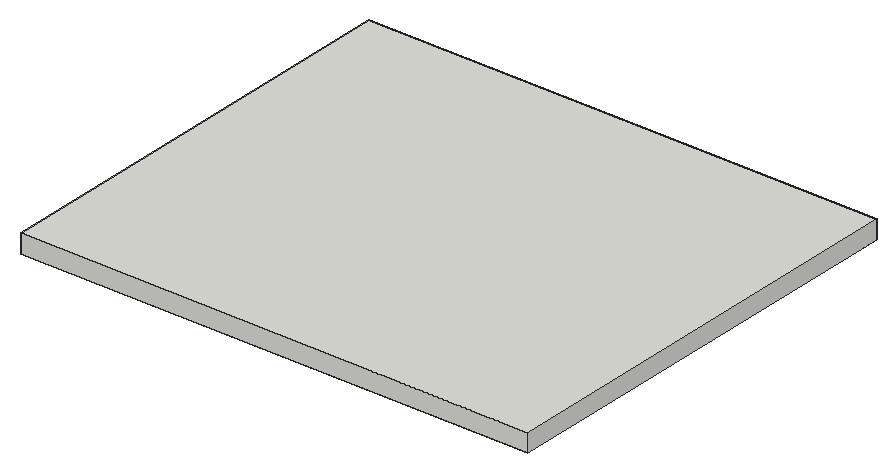
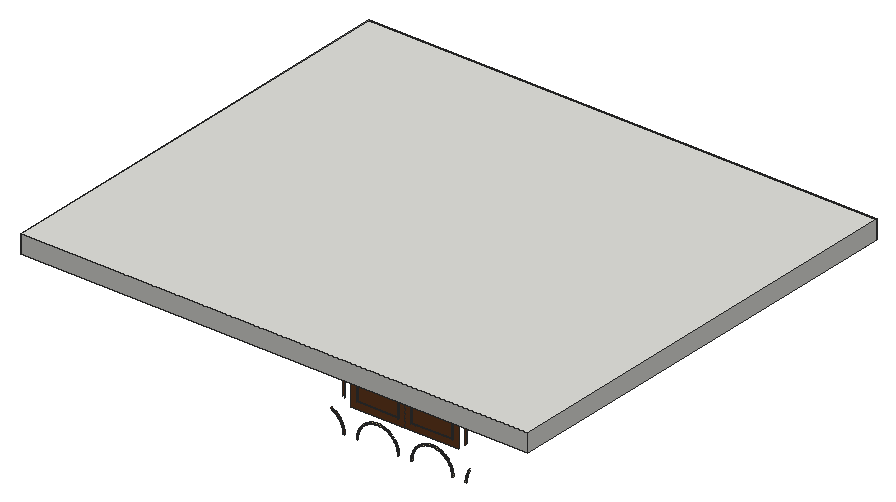
# SketchUp Ruby script. Lengths in inches.
U = 1.inch
M = Sketchup.active_model
def pt(a) = Geom::Point3d.new(a.map { |v| v * U })
def face(e, loops, mat)
  f = e.add_face(loops[0].map { |a| pt(a) })
  loops[1..].each { |l| e.add_face(l.map { |a| pt(a) }).erase! }
  f.material = f.back_material = mat if mat
  f
end
# faces: each face lists its corners as indices into pts; further lists are holes
def faces(e, pts, list, mat = nil) = list.each { |f| face(e, (f[0].is_a?(Array) ? f : [f]).map { |l| l.map { |i| pts[i] } }, mat) }
# xy, xz, yz: faces in a plane at the given z, y or x. An outline is a flat list of corners, or four numbers for a rectangle; further outlines are holes
def ring(l) = l.size == 4 ? [[l[0], l[1]], [l[2], l[1]], [l[2], l[3]], [l[0], l[3]]] : l.each_slice(2).to_a
def flat(e, list, mat, &to3) = list.each { |f| face(e, (f[0].is_a?(Array) ? f : [f]).map { |l| ring(l).map { |u, v| to3.(u, v) } }, mat) }
def xy(e, z, list, mat = nil) = flat(e, list, mat) { |x, y| [x, y, z] }
def xz(e, y, list, mat = nil) = flat(e, list, mat) { |x, z| [x, y, z] }
def yz(e, x, list, mat = nil) = flat(e, list, mat) { |y, z| [x, y, z] }
def lines(e, pts, list) = list.each { |a, b| e.add_line(pt(pts[a]), pt(pts[b])) }
# prism: a flat outline (further loops are holes) pulled along v
def prism(e, loops, v, mat = nil)
  f = face(e, loops, mat); d = Geom::Vector3d.new(v.map { |x| x * U })
  f.pushpull(f.normal.samedirection?(d) ? d.length : -d.length)
end
def box(e, o, s, mat = nil) = prism(e, [[o, [o[0] + s[0], o[1], o[2]], [o[0] + s[0], o[1] + s[1], o[2]], [o[0], o[1] + s[1], o[2]]]], [0, 0, s[2]], mat)
def at(x, y, z, deg = 0) = Geom::Transformation.translation(pt([x, y, z])) * Geom::Transformation.rotation(ORIGIN, Z_AXIS, deg.degrees)
def axes(o, x, y, z) = Geom::Transformation.new([*x, 0, *y, 0, *z, 0, *pt(o).to_a, 1])
def part(name) = M.definitions.add(name)
# library, detail: a bought-in or finely detailed component or shape, given as its bounding box
def library(name, o, s) = part(name).tap { |d| box(d.entities, o, s) }
def detail(e, o, s) = box(e.add_group.entities, o, s)
def put(e, d, t, mat = nil) = e.add_instance(d, t).tap { |i| i.material = mat if mat }
def group(e, t, mat = nil) = e.add_group.tap { |g| g.transformation = t; g.material = mat if mat }.entities
root = M.entities
M.materials.add("138_plaster painted wall texture-seamless").color = [214, 198, 153]
M.materials.add("[Wood Veneer 01]").color = [104, 60, 32]
c1 = part("Recessed ceiling light")
xy(c1.entities,0,[[4,0,2.96,0.14,2,0.54,1.17,1.17,0.54,2,0.14,2.96,0,4,0.14,5.04,0.54,6,1.17,6.83,2,7.46,2.96,7.86,4,8,5.04,7.86,6,7.46,6.83,6.83,7.46,6,7.86,5.04,8,4,7.86,2.96,7.46,2,6.83,1.17,6,0.54,5.04,0.14]])
xy(c1.entities,0.2,[[[4,0,5.04,0.14,6,0.54,6.83,1.17,7.46,2,7.86,2.96,8,4,7.86,5.04,7.46,6,6.83,6.83,6,7.46,5.04,7.86,4,8,2.96,7.86,2,7.46,1.17,6.83,0.54,6,0.14,5.04,0,4,0.14,2.96,0.54,2,1.17,1.17,2,0.54,2.96,0.14],[4,0.6,3.12,0.72,2.3,1.06,1.6,1.6,1.06,2.3,0.72,3.12,0.6,4,0.72,4.88,1.06,5.7,1.6,6.4,2.3,6.94,3.12,7.28,4,7.4,4.88,7.28,5.7,6.94,6.4,6.4,6.94,5.7,7.28,4.88,7.4,4,7.28,3.12,6.94,2.3,6.4,1.6,5.7,1.06,4.88,0.72]],[4,0.6,4.88,0.72,5.7,1.06,6.4,1.6,6.94,2.3,7.28,3.12,7.4,4,7.28,4.88,6.94,5.7,6.4,6.4,5.7,6.94,4.88,7.28,4,7.4,3.12,7.28,2.3,6.94,1.6,6.4,1.06,5.7,0.72,4.88,0.6,4,0.72,3.12,1.06,2.3,1.6,1.6,2.3,1.06,3.12,0.72]])
p = [[2.96,0.14,0],[4,0,0],[4,0,0.2],[2.96,0.14,0.2],[5.04,0.14,0],[5.04,0.14,0.2],
  [2,0.54,0],[2,0.54,0.2],[6,0.54,0],[6,0.54,0.2],[1.17,1.17,0],[1.17,1.17,0.2],
  [6.83,1.17,0],[6.83,1.17,0.2],[0.54,2,0],[0.54,2,0.2],[7.46,2,0],[7.46,2,0.2],
  [0.14,2.96,0],[0.14,2.96,0.2],[7.86,2.96,0],[7.86,2.96,0.2],[0,4,0],[0,4,0.2],
  [8,4,0],[8,4,0.2],[0.14,5.04,0],[0.14,5.04,0.2],[7.86,5.04,0],[7.86,5.04,0.2],
  [0.54,6,0],[0.54,6,0.2],[7.46,6,0],[7.46,6,0.2],[1.17,6.83,0],[1.17,6.83,0.2],
  [6.83,6.83,0],[6.83,6.83,0.2],[2,7.46,0],[2,7.46,0.2],[6,7.46,0],[6,7.46,0.2],
  [2.96,7.86,0],[2.96,7.86,0.2],[5.04,7.86,0],[5.04,7.86,0.2],[4,8,0],[4,8,0.2]]
faces(c1.entities,p,[[0,1,2,3],[1,4,5,2],[6,0,3,7],[4,8,9,5],[10,6,7,11],[8,12,13,9],[14,10,11,15],[12,16,17,13],
  [18,14,15,19],[16,20,21,17],[22,18,19,23],[20,24,25,21],[26,22,23,27],[24,28,29,25],[30,26,27,31],[28,32,33,29],
  [34,30,31,35],[32,36,37,33],[38,34,35,39],[36,40,41,37],[42,38,39,43],[40,44,45,41],[46,42,43,47],[44,46,47,45]])
c2 = part("Ceiling panel")
xy(c2.entities,0,[[0,0,0,144,168,144,168,120,24,120,24,24,168,24,168,0],[24,24,168,120]])
xy(c2.entities,6,[[0,0,168,144]])
xz(c2.entities,0,[[0,0,168,6]])
xz(c2.entities,144,[[0,0,168,6]])
yz(c2.entities,0,[[0,0,144,6]])
yz(c2.entities,168,[[0,0,144,6]])
xy(root,90,[[44,119.8,58,120],[62,119.8,76,120]],"[Wood Veneer 01]")
xy(root,90.4,[[44.4,119.8,57.6,120],[62.4,119.8,75.6,120]],"[Wood Veneer 01]")
xy(root,109.6,[[44.4,119.8,57.6,120],[62.4,119.8,75.6,120]],"[Wood Veneer 01]")
xy(root,110,[[44,119.8,58,120],[62,119.8,76,120]],"[Wood Veneer 01]")
xz(root,119.8,[[[44,90,58,110],[44.4,90.4,57.6,109.6]],[[62,90,76,110],[62.4,90.4,75.6,109.6]]],"[Wood Veneer 01]")
xz(root,120,[[[42,88,60,112],[44,90,58,110]],[[60,88,78,112],[62,90,76,110]],[44.4,90.4,57.6,109.6],[62.4,90.4,75.6,109.6]],"[Wood Veneer 01]")
yz(root,39.6,[[119.8,90.4,120,109.6]],"[Wood Veneer 01]")
yz(root,40,[[119.8,90,120,110]],"[Wood Veneer 01]")
yz(root,44,[[119.8,90,120,110]],"[Wood Veneer 01]")
yz(root,44.4,[[119.8,90.4,120,109.6]],"[Wood Veneer 01]")
yz(root,57.6,[[119.8,90.4,120,109.6]],"[Wood Veneer 01]")
yz(root,58,[[119.8,90,120,110]],"[Wood Veneer 01]")
yz(root,62,[[119.8,90,120,110]],"[Wood Veneer 01]")
yz(root,62.4,[[119.8,90.4,120,109.6]],"[Wood Veneer 01]")
yz(root,75.6,[[119.8,90.4,120,109.6]],"[Wood Veneer 01]")
yz(root,76,[[119.8,90,120,110]],"[Wood Veneer 01]")
yz(root,80,[[119.8,90,120,110]],"[Wood Veneer 01]")
yz(root,80.4,[[119.8,90.4,120,109.6]],"[Wood Veneer 01]")
p = [[39.59,120,79.43],[39.6,120,79],[39.6,119.8,79],[39.59,119.8,79.43],[40,120,79],[39.99,120,79.46],
  [39.99,119.8,79.46],[40,119.8,79],[44.01,120,79.46],[44,120,79],[44,119.8,79],[44.01,119.8,79.46],
  [44.4,120,79],[44.41,120,79.43],[44.41,119.8,79.43],[44.4,119.8,79],[57.59,120,79.43],[57.6,120,79],
  [57.6,119.8,79],[57.59,119.8,79.43],[58,120,79],[57.99,120,79.46],[57.99,119.8,79.46],[58,119.8,79],
  [62.01,120,79.46],[62,120,79],[62,119.8,79],[62.01,119.8,79.46],[62.4,120,79],[62.41,120,79.43],
  [62.41,119.8,79.43],[62.4,119.8,79],[75.59,120,79.43],[75.6,120,79],[75.6,119.8,79],[75.59,119.8,79.43],
  [76,120,79],[75.99,120,79.46],[75.99,119.8,79.46],[76,119.8,79],[80.01,120,79.46],[80,120,79],
  [80,119.8,79],[80.01,119.8,79.46],[80.4,120,79],[80.41,120,79.43],[80.41,119.8,79.43],[80.4,119.8,79],
  [39.54,120,79.86],[39.54,119.8,79.86],[44.46,120,79.86],[44.46,119.8,79.86],[57.54,120,79.86],[57.54,119.8,79.86],
  [62.46,120,79.86],[62.46,119.8,79.86],[75.54,120,79.86],[75.54,119.8,79.86],[80.46,120,79.86],[80.46,119.8,79.86],
  [39.94,120,79.91],[39.94,119.8,79.91],[44.06,120,79.91],[44.06,119.8,79.91],[57.94,120,79.91],[57.94,119.8,79.91],
  [62.06,120,79.91],[62.06,119.8,79.91],[75.94,120,79.91],[75.94,119.8,79.91],[80.06,120,79.91],[80.06,119.8,79.91],
  [39.47,120,80.29],[39.47,119.8,80.29],[39.87,120,80.37],[39.87,119.8,80.37],[44.13,120,80.37],[44.13,119.8,80.37],
  [44.53,120,80.29],[44.53,119.8,80.29],[57.47,120,80.29],[57.47,119.8,80.29],[57.87,120,80.37],[57.87,119.8,80.37],
  [62.13,120,80.37],[62.13,119.8,80.37],[62.53,120,80.29],[62.53,119.8,80.29],[75.47,120,80.29],[75.47,119.8,80.29],
  [75.87,120,80.37],[75.87,119.8,80.37],[80.13,120,80.37],[80.13,119.8,80.37],[80.53,120,80.29],[80.53,119.8,80.29],
  [39.375,120,80.71],[39.375,119.8,80.71],[44.625,120,80.71],[44.625,119.8,80.71],[57.375,120,80.71],[57.375,119.8,80.71],
  [62.625,120,80.71],[62.625,119.8,80.71],[75.375,120,80.71],[75.375,119.8,80.71],[80.625,120,80.71],[80.625,119.8,80.71],
  [39.76,120,80.8125],[39.76,119.8,80.8125],[44.24,120,80.8125],[44.24,119.8,80.8125],[57.76,120,80.8125],[57.76,119.8,80.8125],
  [62.24,120,80.8125],[62.24,119.8,80.8125],[75.76,120,80.8125],[75.76,119.8,80.8125],[80.24,120,80.8125],[80.24,119.8,80.8125],
  [39.25,120,81.12],[39.25,119.8,81.12],[44.75,120,81.12],[44.75,119.8,81.12],[57.25,120,81.12],[57.25,119.8,81.12],
  [62.75,120,81.12],[62.75,119.8,81.12],[75.25,120,81.12],[75.25,119.8,81.12],[80.75,120,81.12],[80.75,119.8,81.12],
  [39.63,120,81.25],[39.63,119.8,81.25],[44.37,120,81.25],[44.37,119.8,81.25],[57.63,120,81.25],[57.63,119.8,81.25],
  [62.37,120,81.25],[62.37,119.8,81.25],[75.63,120,81.25],[75.63,119.8,81.25],[80.37,120,81.25],[80.37,119.8,81.25],
  [39.1,120,81.53],[39.1,119.8,81.53],[44.9,120,81.53],[44.9,119.8,81.53],[57.1,120,81.53],[57.1,119.8,81.53],
  [62.9,120,81.53],[62.9,119.8,81.53],[75.1,120,81.53],[75.1,119.8,81.53],[80.9,120,81.53],[80.9,119.8,81.53],
  [39.47,120,81.68],[39.47,119.8,81.68],[44.53,120,81.68],[44.53,119.8,81.68],[57.47,120,81.68],[57.47,119.8,81.68],
  [62.53,120,81.68],[62.53,119.8,81.68],[75.47,120,81.68],[75.47,119.8,81.68],[80.53,120,81.68],[80.53,119.8,81.68],
  [38.92,120,81.92],[38.92,119.8,81.92],[45.08,120,81.92],[45.08,119.8,81.92],[56.92,120,81.92],[56.92,119.8,81.92],
  [63.08,120,81.92],[63.08,119.8,81.92],[74.92,120,81.92],[74.92,119.8,81.92],[81.08,120,81.92],[81.08,119.8,81.92],
  [39.28,120,82.1],[39.28,119.8,82.1],[44.72,120,82.1],[44.72,119.8,82.1],[57.28,120,82.1],[57.28,119.8,82.1],
  [62.72,120,82.1],[62.72,119.8,82.1],[75.28,120,82.1],[75.28,119.8,82.1],[80.72,120,82.1],[80.72,119.8,82.1],
  [38.72,120,82.3],[38.72,119.8,82.3],[45.28,120,82.3],[45.28,119.8,82.3],[56.72,120,82.3],[56.72,119.8,82.3],
  [63.28,120,82.3],[63.28,119.8,82.3],[74.72,120,82.3],[74.72,119.8,82.3],[81.28,120,82.3],[81.28,119.8,82.3],
  [39.0625,120,82.5],[39.0625,119.8,82.5],[44.9375,120,82.5],[44.9375,119.8,82.5],[57.0625,120,82.5],[57.0625,119.8,82.5],
  [62.9375,120,82.5],[62.9375,119.8,82.5],[75.0625,120,82.5],[75.0625,119.8,82.5],[80.9375,120,82.5],[80.9375,119.8,82.5],
  [38.49,120,82.67],[38.49,119.8,82.67],[45.51,120,82.67],[45.51,119.8,82.67],[56.49,120,82.67],[56.49,119.8,82.67],
  [63.51,120,82.67],[63.51,119.8,82.67],[74.49,120,82.67],[74.49,119.8,82.67],[81.51,120,82.67],[81.51,119.8,82.67],
  [38.82,120,82.89],[38.82,119.8,82.89],[45.18,120,82.89],[45.18,119.8,82.89],[56.82,120,82.89],[56.82,119.8,82.89],
  [63.18,120,82.89],[63.18,119.8,82.89],[74.82,120,82.89],[74.82,119.8,82.89],[81.18,120,82.89],[81.18,119.8,82.89],
  [45.76,120,83.02],[45.76,119.8,83.02],[56.24,120,83.02],[56.24,119.8,83.02],[63.76,120,83.02],[63.76,119.8,83.02],
  [74.24,120,83.02],[74.24,119.8,83.02],[81.76,120,83.02],[81.76,119.8,83.02],[38.55,120,83.26],[38.55,119.8,83.26],
  [45.45,120,83.26],[45.45,119.8,83.26],[56.55,120,83.26],[56.55,119.8,83.26],[63.45,120,83.26],[63.45,119.8,83.26],
  [74.55,120,83.26],[74.55,119.8,83.26],[81.45,120,83.26],[81.45,119.8,83.26],[46.04,120,83.35],[46.04,119.8,83.35],
  [55.96,120,83.35],[55.96,119.8,83.35],[64.04,120,83.35],[64.04,119.8,83.35],[73.96,120,83.35],[73.96,119.8,83.35],
  [82.04,120,83.35],[82.04,119.8,83.35],[45.74,120,83.62],[45.74,119.8,83.62],[56.26,120,83.62],[56.26,119.8,83.62],
  [63.74,120,83.62],[63.74,119.8,83.62],[74.26,120,83.62],[74.26,119.8,83.62],[81.74,120,83.62],[81.74,119.8,83.62],
  [46.33,120,83.67],[46.33,119.8,83.67],[55.67,120,83.67],[55.67,119.8,83.67],[64.33,120,83.67],[64.33,119.8,83.67],
  [73.67,120,83.67],[73.67,119.8,83.67],[82.33,120,83.67],[82.33,119.8,83.67],[46.05,120,83.95],[46.05,119.8,83.95],
  [55.95,120,83.95],[55.95,119.8,83.95],[64.05,120,83.95],[64.05,119.8,83.95],[73.95,120,83.95],[73.95,119.8,83.95],
  [82.05,120,83.95],[82.05,119.8,83.95],[46.65,120,83.96],[46.65,119.8,83.96],[55.35,120,83.96],[55.35,119.8,83.96],
  [64.65,120,83.96],[64.65,119.8,83.96],[73.35,120,83.96],[73.35,119.8,83.96],[82.65,120,83.96],[82.65,119.8,83.96],
  [46.38,120,84.26],[46.38,119.8,84.26],[55.62,120,84.26],[55.62,119.8,84.26],[64.38,120,84.26],[64.38,119.8,84.26],
  [73.62,120,84.26],[73.62,119.8,84.26],[82.38,120,84.26],[82.38,119.8,84.26],[46.98,120,84.24],[46.98,119.8,84.24],
  [55.02,120,84.24],[55.02,119.8,84.24],[64.98,120,84.24],[64.98,119.8,84.24],[73.02,120,84.24],[73.02,119.8,84.24],
  [82.98,120,84.24],[82.98,119.8,84.24],[47.33,120,84.49],[47.33,119.8,84.49],[54.67,120,84.49],[54.67,119.8,84.49],
  [65.33,120,84.49],[65.33,119.8,84.49],[72.67,120,84.49],[72.67,119.8,84.49],[83.33,120,84.49],[83.33,119.8,84.49],
  [46.74,120,84.55],[46.74,119.8,84.55],[55.26,120,84.55],[55.26,119.8,84.55],[64.74,120,84.55],[64.74,119.8,84.55],
  [73.26,120,84.55],[73.26,119.8,84.55],[82.74,120,84.55],[82.74,119.8,84.55],[47.7,120,84.72],[47.7,119.8,84.72],
  [54.3,120,84.72],[54.3,119.8,84.72],[65.7,120,84.72],[65.7,119.8,84.72],[72.3,120,84.72],[72.3,119.8,84.72],
  [83.7,120,84.72],[83.7,119.8,84.72],[47.11,120,84.82],[47.11,119.8,84.82],[54.89,120,84.82],[54.89,119.8,84.82],
  [65.11,120,84.82],[65.11,119.8,84.82],[72.89,120,84.82],[72.89,119.8,84.82],[83.11,120,84.82],[83.11,119.8,84.82],
  [48.08,120,84.92],[48.08,119.8,84.92],[53.92,120,84.92],[53.92,119.8,84.92],[66.08,120,84.92],[66.08,119.8,84.92],
  [71.92,120,84.92],[71.92,119.8,84.92],[84.08,120,84.92],[84.08,119.8,84.92],[47.5,120,85.0625],[47.5,119.8,85.0625],
  [54.5,120,85.0625],[54.5,119.8,85.0625],[65.5,120,85.0625],[65.5,119.8,85.0625],[72.5,120,85.0625],[72.5,119.8,85.0625],
  [83.5,120,85.0625],[83.5,119.8,85.0625],[48.47,120,85.1],[48.47,119.8,85.1],[53.53,120,85.1],[53.53,119.8,85.1],
  [66.47,120,85.1],[66.47,119.8,85.1],[71.53,120,85.1],[71.53,119.8,85.1],[47.9,120,85.28],[47.9,119.8,85.28],
  [48.88,120,85.25],[48.88,119.8,85.25],[53.12,120,85.25],[53.12,119.8,85.25],[54.1,120,85.28],[54.1,119.8,85.28],
  [65.9,120,85.28],[65.9,119.8,85.28],[66.88,120,85.25],[66.88,119.8,85.25],[71.12,120,85.25],[71.12,119.8,85.25],
  [72.1,120,85.28],[72.1,119.8,85.28],[83.9,120,85.28],[83.9,119.8,85.28],[49.29,120,85.375],[49.29,119.8,85.375],
  [52.71,120,85.375],[52.71,119.8,85.375],[67.29,120,85.375],[67.29,119.8,85.375],[70.71,120,85.375],[70.71,119.8,85.375],
  [48.32,120,85.47],[48.32,119.8,85.47],[53.68,120,85.47],[53.68,119.8,85.47],[66.32,120,85.47],[66.32,119.8,85.47],
  [71.68,120,85.47],[71.68,119.8,85.47],[84.32,120,85.47],[84.32,119.8,85.47],[49.71,120,85.47],[49.71,119.8,85.47],
  [52.29,120,85.47],[52.29,119.8,85.47],[67.71,120,85.47],[67.71,119.8,85.47],[70.29,120,85.47],[70.29,119.8,85.47],
  [48.75,120,85.63],[48.75,119.8,85.63],[50.14,120,85.54],[50.14,119.8,85.54],[50.57,120,85.59],[50.57,119.8,85.59],
  [51.43,120,85.59],[51.86,120,85.54],[51.86,119.8,85.54],[51.43,119.8,85.59],[53.25,120,85.63],[53.25,119.8,85.63],
  [66.75,120,85.63],[66.75,119.8,85.63],[68.14,120,85.54],[68.14,119.8,85.54],[68.57,120,85.59],[68.57,119.8,85.59],
  [69.43,120,85.59],[69.86,120,85.54],[69.86,119.8,85.54],[69.43,119.8,85.59],[71.25,120,85.63],[71.25,119.8,85.63],
  [49.1875,120,85.76],[49.1875,119.8,85.76],[51,120,85.6],[51,119.8,85.6],[52.8125,120,85.76],[52.8125,119.8,85.76],
  [67.1875,120,85.76],[67.1875,119.8,85.76],[69,120,85.6],[69,119.8,85.6],[70.8125,120,85.76],[70.8125,119.8,85.76],
  [49.63,120,85.87],[49.63,119.8,85.87],[52.37,120,85.87],[52.37,119.8,85.87],[67.63,120,85.87],[67.63,119.8,85.87],
  [70.37,120,85.87],[70.37,119.8,85.87],[50.09,120,85.94],[50.09,119.8,85.94],[50.54,120,85.99],[50.54,119.8,85.99],
  [51.91,120,85.94],[51.46,120,85.99],[51.46,119.8,85.99],[51.91,119.8,85.94],[68.09,120,85.94],[68.09,119.8,85.94],
  [68.54,120,85.99],[68.54,119.8,85.99],[69.91,120,85.94],[69.46,120,85.99],[69.46,119.8,85.99],[69.91,119.8,85.94],
  [51,120,86],[51,119.8,86],[69,120,86],[69,119.8,86]]
faces(root,p,[[0,1,2,3],[4,5,6,7],[8,9,10,11],[12,13,14,15],[16,17,18,19],[20,21,22,23],[24,25,26,27],[28,29,30,31],
  [32,33,34,35],[36,37,38,39],[48,0,3,49],[13,50,51,14],[52,16,19,53],[29,54,55,30],[56,32,35,57],[5,60,61,6],
  [62,8,11,63],[21,64,65,22],[66,24,27,67],[37,68,69,38],[72,48,49,73],[60,74,75,61],[76,62,63,77],[50,78,79,51],
  [80,52,53,81],[64,82,83,65],[84,66,67,85],[54,86,87,55],[88,56,57,89],[68,90,91,69],[96,72,73,97],[78,98,99,79],
  [100,80,81,101],[86,102,103,87],[104,88,89,105],[74,108,109,75],[110,76,77,111],[82,112,113,83],[114,84,85,115],[90,116,117,91],
  [120,96,97,121],[98,122,123,99],[124,100,101,125],[102,126,127,103],[128,104,105,129],[108,132,133,109],[134,110,111,135],[112,136,137,113],
  [138,114,115,139],[116,140,141,117],[144,120,121,145],[122,146,147,123],[148,124,125,149],[126,150,151,127],[152,128,129,153],[132,156,157,133],
  [158,134,135,159],[136,160,161,137],[162,138,139,163],[140,164,165,141],[168,144,145,169],[146,170,171,147],[172,148,149,173],[150,174,175,151],
  [176,152,153,177],[156,180,181,157],[182,158,159,183],[160,184,185,161],[186,162,163,187],[164,188,189,165],[192,168,169,193],[170,194,195,171],
  [196,172,173,197],[174,198,199,175],[200,176,177,201],[180,204,205,181],[206,182,183,207],[184,208,209,185],[210,186,187,211],[188,212,213,189],
  [216,192,193,217],[194,218,219,195],[220,196,197,221],[198,222,223,199],[224,200,201,225],[204,228,229,205],[230,206,207,231],[208,232,233,209],
  [234,210,211,235],[212,236,237,213],[218,240,241,219],[242,220,221,243],[222,244,245,223],[246,224,225,247],[228,250,251,229],[252,230,231,253],
  [232,254,255,233],[256,234,235,257],[236,258,259,237],[240,262,263,241],[264,242,243,265],[244,266,267,245],[268,246,247,269],[272,252,253,273],
  [254,274,275,255],[276,256,257,277],[258,278,279,259],[262,282,283,263],[284,264,265,285],[266,286,287,267],[288,268,269,289],[292,272,273,293],
  [274,294,295,275],[296,276,277,297],[278,298,299,279],[282,302,303,283],[304,284,285,305],[286,306,307,287],[308,288,289,309],[312,292,293,313],
  [294,314,315,295],[316,296,297,317],[298,318,319,299],[302,322,323,303],[324,304,305,325],[306,326,327,307],[328,308,309,329],[322,332,333,323],
  [334,324,325,335],[326,336,337,327],[338,328,329,339],[342,312,313,343],[314,344,345,315],[346,316,317,347],[318,348,349,319],[332,352,353,333],
  [354,334,335,355],[336,356,357,337],[358,338,339,359],[362,342,343,363],[344,364,365,345],[366,346,347,367],[348,368,369,349],[352,372,373,353],
  [374,354,355,375],[356,376,377,357],[378,358,359,379],[382,362,363,383],[364,384,385,365],[386,366,367,387],[368,388,389,369],[372,392,393,373],
  [394,374,375,395],[376,396,397,377],[398,378,379,399],[400,382,383,401],[392,402,403,393],[404,394,395,405],[384,406,407,385],[408,386,387,409],
  [396,410,411,397],[412,398,399,413],[388,414,415,389],[402,418,419,403],[420,404,405,421],[410,422,423,411],[424,412,413,425],[426,400,401,427],
  [406,428,429,407],[430,408,409,431],[414,432,433,415],[418,436,437,419],[438,420,421,439],[422,440,441,423],[442,424,425,443],[444,426,427,445],
  [436,446,447,437],[446,448,449,447],[450,451,452,453],[451,438,439,452],[428,454,455,429],[456,430,431,457],[440,458,459,441],[458,460,461,459],
  [462,463,464,465],[463,442,443,464],[432,466,467,433],[468,444,445,469],[448,470,471,449],[470,450,453,471],[454,472,473,455],[474,456,457,475],
  [460,476,477,461],[476,462,465,477],[466,478,479,467],[480,468,469,481],[472,482,483,473],[484,474,475,485],[478,486,487,479],[488,480,481,489],
  [490,488,489,491],[492,493,494,495],[482,492,495,483],[496,484,485,497],[498,496,497,499],[500,501,502,503],[486,500,503,487],[504,490,491,505],
  [493,504,505,494],[506,498,499,507],[501,506,507,502]],"138_plaster painted wall texture-seamless")
faces(root,p,[[40,41,42,43],[44,45,46,47],[45,58,59,46],[70,40,43,71],[92,70,71,93],[58,94,95,59],[94,106,107,95],[118,92,93,119],
  [106,130,131,107],[142,118,119,143],[130,154,155,131],[166,142,143,167],[154,178,179,155],[190,166,167,191],[178,202,203,179],[214,190,191,215],
  [202,226,227,203],[238,214,215,239],[226,248,249,227],[260,238,239,261],[248,270,271,249],[280,260,261,281],[270,290,291,271],[300,280,281,301],
  [290,310,311,291],[320,300,301,321],[310,330,331,311],[330,340,341,331],[350,320,321,351],[340,360,361,341],[370,350,351,371],[360,380,381,361],
  [390,370,371,391],[416,390,391,417],[434,416,417,435]],"[Wood Veneer 01]")
g1 = group(root,at(0,0,118.2))
put(g1,c1,axes([92,68,-6],[1,0,0],[0,1,0],[0,0,-1]))
put(g1,c1,axes([92,92,-6],[1,0,0],[0,1,0],[0,0,-1]))
put(g1,c1,axes([44,44,-6],[1,0,0],[0,1,0],[0,0,-1]))
put(g1,c1,axes([140,92,-6],[1,0,0],[0,1,0],[0,0,-1]))
put(g1,c1,axes([92,44,-6],[1,0,0],[0,1,0],[0,0,-1]))
put(g1,c1,axes([140,44,-6],[1,0,0],[0,1,0],[0,0,-1]))
put(g1,c2,axes([0,144,-6],[1,0,0],[0,-1,0],[0,0,1]))
put(g1,c1,axes([116,68,-6],[1,0,0],[0,1,0],[0,0,-1]))
put(g1,c1,axes([44,92,-6],[1,0,0],[0,1,0],[0,0,-1]))
